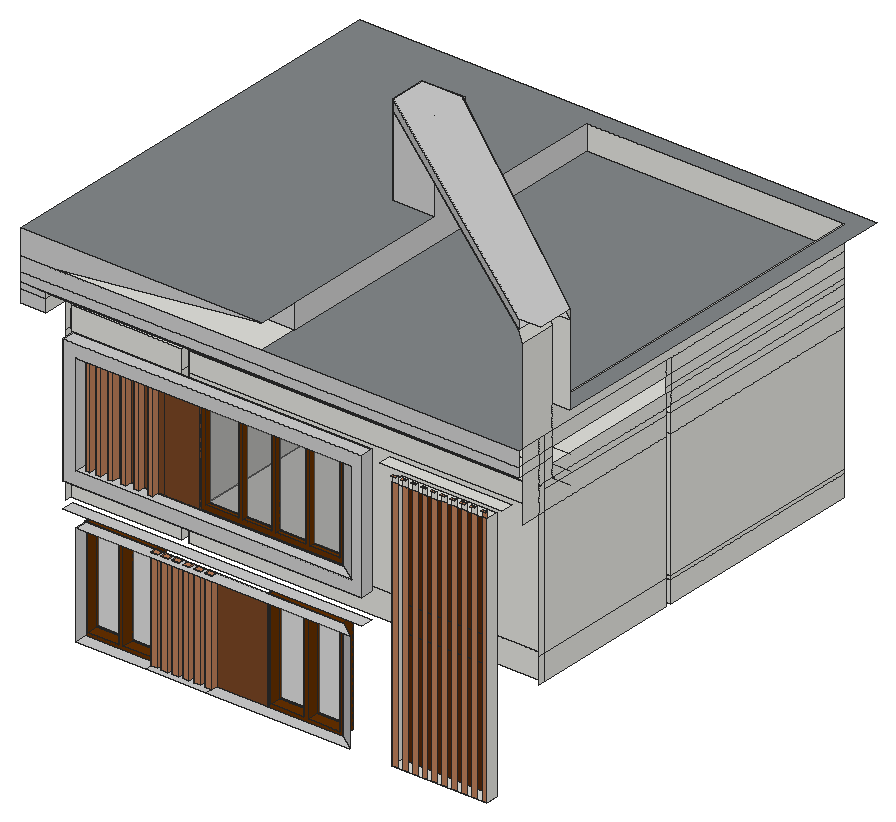
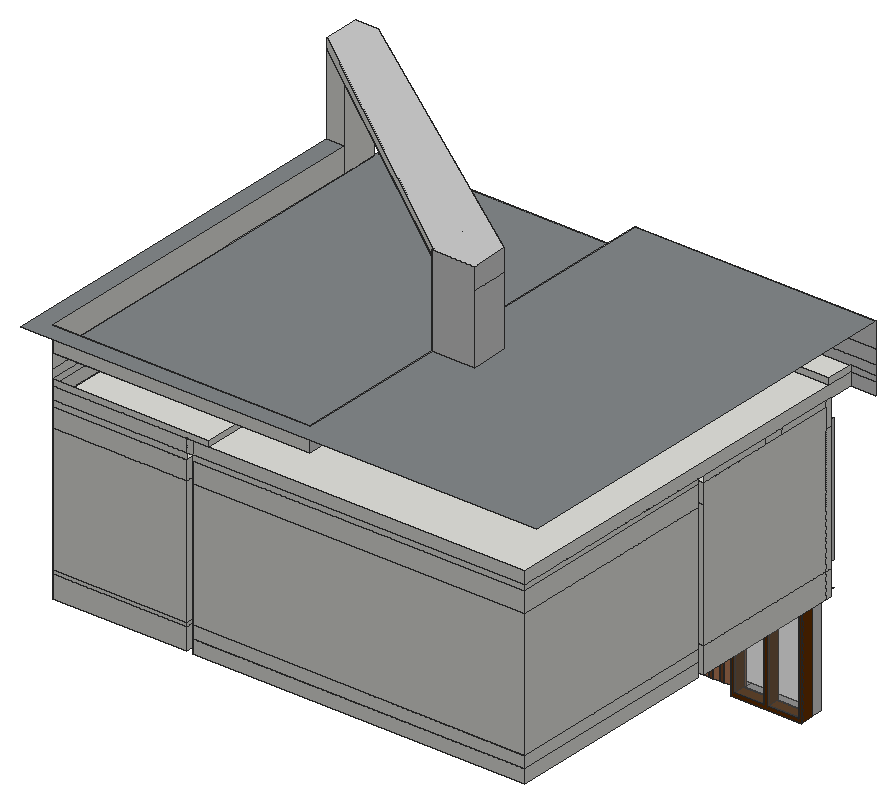
# SketchUp Ruby script. Lengths in inches.
U = 1.inch
M = Sketchup.active_model
def pt(a) = Geom::Point3d.new(a.map { |v| v * U })
def face(e, loops, mat)
  f = e.add_face(loops[0].map { |a| pt(a) })
  loops[1..].each { |l| e.add_face(l.map { |a| pt(a) }).erase! }
  f.material = f.back_material = mat if mat
  f
end
# faces: each face lists its corners as indices into pts; further lists are holes
def faces(e, pts, list, mat = nil) = list.each { |f| face(e, (f[0].is_a?(Array) ? f : [f]).map { |l| l.map { |i| pts[i] } }, mat) }
# xy, xz, yz: faces in a plane at the given z, y or x. An outline is a flat list of corners, or four numbers for a rectangle; further outlines are holes
def ring(l) = l.size == 4 ? [[l[0], l[1]], [l[2], l[1]], [l[2], l[3]], [l[0], l[3]]] : l.each_slice(2).to_a
def flat(e, list, mat, &to3) = list.each { |f| face(e, (f[0].is_a?(Array) ? f : [f]).map { |l| ring(l).map { |u, v| to3.(u, v) } }, mat) }
def xy(e, z, list, mat = nil) = flat(e, list, mat) { |x, y| [x, y, z] }
def xz(e, y, list, mat = nil) = flat(e, list, mat) { |x, z| [x, y, z] }
def yz(e, x, list, mat = nil) = flat(e, list, mat) { |y, z| [x, y, z] }
def lines(e, pts, list) = list.each { |a, b| e.add_line(pt(pts[a]), pt(pts[b])) }
# prism: a flat outline (further loops are holes) pulled along v
def prism(e, loops, v, mat = nil)
  f = face(e, loops, mat); d = Geom::Vector3d.new(v.map { |x| x * U })
  f.pushpull(f.normal.samedirection?(d) ? d.length : -d.length)
end
def box(e, o, s, mat = nil) = prism(e, [[o, [o[0] + s[0], o[1], o[2]], [o[0] + s[0], o[1] + s[1], o[2]], [o[0], o[1] + s[1], o[2]]]], [0, 0, s[2]], mat)
def at(x, y, z, deg = 0) = Geom::Transformation.translation(pt([x, y, z])) * Geom::Transformation.rotation(ORIGIN, Z_AXIS, deg.degrees)
def axes(o, x, y, z) = Geom::Transformation.new([*x, 0, *y, 0, *z, 0, *pt(o).to_a, 1])
def part(name) = M.definitions.add(name)
# library, detail: a bought-in or finely detailed component or shape, given as its bounding box
def library(name, o, s) = part(name).tap { |d| box(d.entities, o, s) }
def detail(e, o, s) = box(e.add_group.entities, o, s)
def put(e, d, t, mat = nil) = e.add_instance(d, t).tap { |i| i.material = mat if mat }
def group(e, t, mat = nil) = e.add_group.tap { |g| g.transformation = t; g.material = mat if mat }.entities
root = M.entities
M.materials.add("[Blacktop Old 01]").color = [132, 136, 139]
M.materials.add("[Brick Antique 01]").color = [88, 41, 11]
M.materials.add("[Carrera Marble]").color = [207, 207, 207]
M.materials.add("[Color A08]").color = [102, 48, 0]
M.materials.add("[Translucent Glass Gray]").color = [128, 128, 128]
M.materials["[Translucent Glass Gray]"].alpha = 0.5
M.materials.add("[Wood Veneer 01]").color = [120, 70, 37]
M.materials.add("[Wood Veneer 02]").color = [190, 128, 91]
c1 = part("Group\#1")
xy(c1.entities,0,[[0,0,125.5,0.3125],[0,0.3125,125.5,4]],"[Color A08]")
xy(c1.entities,4.91,[[4.91,0,60.47,0.3125],[60.47,0,67.75,0.3125],[67.75,0,120.59,0.3125],[4.91,0.3125,60.47,4],[60.47,0.3125,67.75,4],
  [67.75,0.3125,120.59,4]],"[Color A08]")
xy(c1.entities,153.9,[[4.91,0,60.47,0.3125],[67.75,0,120.59,0.3125],[4.91,0.3125,60.47,4],[67.75,0.3125,120.59,4]],"[Color A08]")
xy(c1.entities,158.8125,[[0,0,125.5,0.3125],[0,0.3125,125.5,4]],"[Color A08]")
xz(c1.entities,0,[[[0,0,125.5,158.8125],[4.91,4.91,4.91,153.9,60.47,153.9,60.47,4.91,67.75,4.91,67.75,153.9,120.59,153.9,120.59,4.91]]],"[Color A08]")
xz(c1.entities,0,[[4.91,4.91,60.47,153.9],[67.75,4.91,120.59,153.9]],"[Translucent Glass Gray]")
xz(c1.entities,0.3125,[[[0,0,125.5,158.8125],[4.91,4.91,4.91,153.9,60.47,153.9,60.47,4.91,67.75,4.91,67.75,153.9,120.59,153.9,120.59,4.91]]],"[Color A08]")
xz(c1.entities,4,[[[0,0,125.5,158.8125],[4.91,4.91,4.91,153.9,60.47,153.9,60.47,4.91,67.75,4.91,67.75,153.9,120.59,153.9,120.59,4.91]]],"[Color A08]")
yz(c1.entities,0,[[0,0,0.3125,158.8125],[0.3125,0,4,158.8125]],"[Color A08]")
yz(c1.entities,4.91,[[0,4.91,0.3125,153.9],[0.3125,4.91,4,153.9]],"[Color A08]")
yz(c1.entities,60.47,[[0,4.91,0.3125,153.9],[0.3125,4.91,4,153.9]],"[Color A08]")
yz(c1.entities,67.75,[[0,4.91,0.3125,153.9],[0.3125,4.91,4,153.9]],"[Color A08]")
yz(c1.entities,120.59,[[0,4.91,0.3125,153.9],[0.3125,4.91,4,153.9]],"[Color A08]")
yz(c1.entities,125.5,[[0,0,0.3125,158.8125],[0.3125,0,4,158.8125]],"[Color A08]")
xy(root,441,[[341.75,90.75,431.1875,102.75],[43.25,102.75,108.92,108.75],[215.87,102.75,285.875,108.75]])
xy(root,441,[[43.25,90.75,108.92,102.75],[108.92,90.75,166.36,90.75,166.36,96.875,159.8,96.875,159.8,102.75,155.92,102.75,155.92,96.875,149.36,96.875,149.36,102.75,145.48,102.75,145.48,96.875,138.92,96.875,138.92,102.75,135.23,102.75,135.23,96.875,128.67,96.875,128.67,102.75,125.36,102.75,125.36,96.875,118.8,96.875,118.8,102.75,115.48,102.75,115.48,96.875,108.92,96.875],[166.36,90.75,301.84,90.75,285.875,102.75,166.36,102.75]],"[Carrera Marble]")
xy(root,441,[[108.92,96.875,115.48,102.75],[118.8,96.875,125.36,102.75],[128.67,96.875,135.23,102.75],[138.92,96.875,145.48,102.75],[149.36,96.875,155.92,102.75],
  [159.8,96.875,166.36,102.75]],"[Wood Veneer 02]")
xy(root,537,[[43.25,102.75,108.92,108.75],[215.87,102.75,285.875,108.75]])
xy(root,537,[[43.25,90.75,43.25,102.75,108.92,102.75,108.92,96.875,115.48,96.875,115.48,102.75,118.8,102.75,118.8,96.875,125.36,96.875,125.36,102.75,128.67,102.75,128.67,96.875,135.23,96.875,135.23,102.75,138.92,102.75,138.92,96.875,145.48,96.875,145.48,102.75,149.36,102.75,149.36,96.875,155.92,96.875,155.92,102.75,159.8,102.75,159.8,96.875,166.36,96.875,166.36,102.75,285.875,102.75,301.84,90.75]],"[Carrera Marble]")
xy(root,537,[[108.92,96.875,115.48,102.75],[118.8,96.875,125.36,102.75],[128.67,96.875,135.23,102.75],[138.92,96.875,145.48,102.75],[149.36,96.875,155.92,102.75],
  [159.8,96.875,166.36,102.75]],"[Wood Veneer 02]")
xy(root,549,[[31.25,90.75,312.9375,102.75]],"[Carrera Marble]")
xy(root,561.75,[[24.5,258.8125,337.8125,463]])
xy(root,569.625,[[343.8125,258.8125,470.5,463]])
xy(root,573,[[24.5,108.75,129.23,252.8125],[135.23,108.75,470.5,252.8125],[24.5,258.8125,337.8125,463],[343.8125,258.8125,470.5,463]])
xy(root,573,[[31.25,90.75,312.9375,102.75]],"[Carrera Marble]")
xy(root,585,[[150.42,102.75,285.875,108.75]])
xy(root,585,[[43.25,90.75,304.01,90.75,285.875,102.75,111.29,102.75,111.29,96.0625,106.64,96.0625,106.64,102.75,98.03,102.75,98.03,96.0625,93.38,96.0625,93.38,102.75,85.91,102.75,85.91,96.0625,81.26,96.0625,81.26,102.75,74.22,102.75,74.22,96.0625,69.57,96.0625,69.57,102.75,62.82,102.75,62.82,96.0625,58.17,96.0625,58.17,102.75,52.63,102.75,52.63,96.0625,47.98,96.0625,47.98,102.75,43.25,102.75]],"[Carrera Marble]")
xy(root,585,[[47.98,96.0625,52.63,102.75],[58.17,96.0625,62.82,102.75],[69.57,96.0625,74.22,102.75],[81.26,96.0625,85.91,102.75],[93.38,96.0625,98.03,102.75],
  [106.64,96.0625,111.29,102.75]],"[Wood Veneer 02]")
xy(root,681,[[341.75,90.75,431.1875,102.75]])
xy(root,681,[[43.25,90.75,43.25,102.75,47.98,102.75,47.98,96.0625,52.63,96.0625,52.63,102.75,58.17,102.75,58.17,96.0625,62.82,96.0625,62.82,102.75,69.57,102.75,69.57,96.0625,74.22,96.0625,74.22,102.75,81.26,102.75,81.26,96.0625,85.91,96.0625,85.91,102.75,93.38,102.75,93.38,96.0625,98.03,96.0625,98.03,102.75,106.64,102.75,106.64,96.0625,111.29,96.0625,111.29,102.75,116.8,102.75,116.8,90.75],[116.8,90.75,150.42,102.75],[150.42,90.75,150.42,102.75,285.875,102.75,304.01,90.75],[150.42,102.75,285.875,108.75]],"[Carrera Marble]")
xy(root,681,[[47.98,96.0625,52.63,102.75],[58.17,96.0625,62.82,102.75],[69.57,96.0625,74.22,102.75],[81.26,96.0625,85.91,102.75],[93.38,96.0625,98.03,102.75],
  [106.64,96.0625,111.29,102.75]],"[Wood Veneer 02]")
xy(root,687.5,[[342.74,88.5,347.3,90.75],[351.99,88.5,356.55,90.75],[361.24,88.5,365.8,90.75],[370.49,88.5,375.05,90.75],[379.74,88.5,384.3,90.75],
  [388.99,88.5,393.55,90.75],[398.24,88.5,402.8,90.75],[407.49,88.5,412.05,90.75],[416.93,88.5,421.49,90.75],[427.11,88.5,431.68,90.75]],"[Wood Veneer 02]")
xy(root,693,[[330,90.75,445.6875,102.75]])
xy(root,693,[[31.25,90.75,312.9375,102.75]],"[Carrera Marble]")
xy(root,711,[[24.5,108.75,129.23,252.8125],[343.8125,258.8125,470.5,463]])
xy(root,712,[[24.5,258.8125,337.8125,463]])
xy(root,717,[[24.5,102.75,470.5,463]])
xy(root,729,[[24.5,104.5625,322.875,463]])
xy(root,734.5625,[[24.5,79.3125,470.5,104.5625]])
xy(root,757.1875,[[28.65,79.3125,227.63,118.3125]])
xy(root,757.1875,[[227.63,79.3125,470.5,463]],"[Blacktop Old 01]")
xy(root,780.4375,[[0,79.3125,227.63,79.3125,227.63,283.73,187.76,283.73,187.76,318.86,227.63,318.86,227.63,463,470.5,463,470.5,118.83,487.5,118.83,487.5,480,0,480]],"[Blacktop Old 01]")
xy(root,856.375,[[466.875,83.875,187.76,283.73,227.63,283.73,227.63,316.62,487.5,118.83,466.875,118.83]],"[Carrera Marble]")
xy(root,865.9375,[[466.875,83.875,487.5,83.875,487.5,118.83,227.63,316.62,227.63,318.86,187.76,318.86,187.76,283.73]],"[Carrera Marble]")
xz(root,79.3125,[[0,717,24.5,729],[0,729,24.5,734.5625],[0,734.5625,470.5,743.3125],[0,743.3125,470.5,757.1875],[0,757.1875,28.65,757.1875,227.63,780.4375,0,780.4375]],"[Carrera Marble]")
xz(root,90.75,[[342.74,681,347.3,687.5],[351.99,681,356.55,687.5],[361.24,681,365.8,687.5],[370.49,681,375.05,687.5],[379.74,681,384.3,687.5],
  [388.99,681,393.55,687.5],[398.24,681,402.8,687.5],[407.49,681,412.05,687.5],[416.93,681,421.49,687.5]])
xz(root,90.75,[[[31.25,573,312.9375,693],[43.25,585,304.01,681]]],"[Carrera Marble]")
xz(root,90.75,[[342.74,441,347.3,681],[351.99,441,356.55,681],[361.24,441,365.8,681],[370.49,441,375.05,681],[379.74,441,384.3,681],
  [388.99,441,393.55,681],[398.24,441,402.8,681],[407.49,441,412.05,681],[416.93,441,421.49,681],[427.11,441,431.1875,681],
  [427.11,681,431.1875,687.5]],"[Wood Veneer 02]")
xz(root,96.0625,[[47.98,585,52.63,681],[58.17,585,62.82,681],[69.57,585,74.22,681],[81.26,585,85.91,681],[93.38,585,98.03,681],
  [106.64,585,111.29,681]],"[Wood Veneer 02]")
xz(root,96.875,[[108.92,441,115.48,537],[118.8,441,125.36,537],[128.67,441,135.23,537],[138.92,441,145.48,537],[149.36,441,155.92,537],
  [159.8,441,166.36,537]],"[Wood Veneer 02]")
xz(root,102.75,[[[31.25,573,312.9375,693],[43.25,585,285.875,681]]])
xz(root,102.75,[[341.75,441,431.1875,549],[341.75,549,431.1875,573],[341.75,573,431.1875,681]],"[Brick Antique 01]")
xz(root,102.75,[[115.48,441,118.8,537],[125.36,441,128.67,537],[135.23,441,138.92,537],[145.48,441,149.36,537],[155.92,441,159.8,537],
  [166.36,441,215.87,537],[43.25,585,47.98,681],[52.63,585,58.17,681],[62.82,585,69.57,681],[74.22,585,81.26,681],
  [85.91,585,93.38,681],[98.03,585,106.64,681],[111.29,585,116.8,681],[116.8,585,150.42,681]],"[Wood Veneer 01]")
xz(root,102.75,[[108.92,441,115.48,537],[118.8,441,125.36,537],[128.67,441,135.23,537],[138.92,441,145.48,537],[149.36,441,155.92,537],
  [159.8,441,166.36,537],[47.98,585,52.63,681],[58.17,585,62.82,681],[69.57,585,74.22,681],[81.26,585,85.91,681],
  [93.38,585,98.03,681],[106.64,585,111.29,681]],"[Wood Veneer 02]")
xz(root,104.5625,[[24.5,729,322.875,734.5625]])
xz(root,108.75,[[24.5,549,129.23,573],[135.23,549,470.5,573],[24.5,573,129.23,711],[[135.23,573,470.5,693],[150.42,585,285.875,681]],[135.23,693,470.5,711]])
xz(root,118.3125,[[28.65,757.1875,227.63,757.1875,227.63,780.4375]],"[Carrera Marble]")
xz(root,118.83,[[470.5,780.4375,470.5,845.4375,466.875,856.375,487.5,856.375,487.5,780.4375]])
xz(root,252.8125,[[24.5,549,129.23,573],[135.23,549,470.5,573],[24.5,573,129.23,693],[135.23,573,470.5,693],[24.5,693,129.23,711]])
xz(root,258.8125,[[24.5,549,337.8125,561.75],[343.8125,549,470.5,569.625],[24.5,561.75,252.45,573],[252.45,561.75,260.7,573],[260.7,561.75,337.8125,573],
  [343.8125,569.625,439.36,573],[439.36,569.625,454.49,573],[454.49,569.625,470.5,573],[24.5,573,337.8125,693],[343.8125,573,470.5,693],
  [24.5,693,337.8125,712],[343.8125,693,470.5,711]])
xz(root,283.73,[[187.76,780.4375,227.63,856.375]],"[Carrera Marble]")
xz(root,318.86,[[187.76,780.4375,227.63,865.9375]],"[Carrera Marble]")
xz(root,463,[[24.5,549,337.8125,561.75],[343.8125,549,470.5,569.625],[24.5,561.75,337.8125,573],[343.8125,569.625,470.5,573],[24.5,573,337.8125,693],
  [343.8125,573,470.5,693],[24.5,693,337.8125,712],[343.8125,693,470.5,711],[343.8125,711,470.5,717],[24.5,712,337.8125,717],
  [24.5,717,337.8125,729],[337.8125,717,343.8125,729],[343.8125,717,470.5,729],[322.875,729,470.5,734.5625],[227.63,757.1875,470.5,780.4375]])
yz(root,24.5,[[102.75,549,108.75,573],[108.75,549,252.8125,573],[258.8125,549,463,561.75],[258.8125,561.75,463,573],[102.75,573,108.75,693],
  [108.75,573,252.8125,711],[258.8125,573,463,693],[102.75,693,108.75,717],[258.8125,693,463,712],[108.75,711,160.04,717],
  [160.04,711,180.78,717],[180.78,711,252.8125,717],[258.8125,712,463,717],[79.3125,717,463,729],[79.3125,729,104.5625,734.5625]])
yz(root,31.25,[[90.75,573,102.75,693]],"[Carrera Marble]")
yz(root,43.25,[[90.75,441,102.75,537],[102.75,441,108.75,537],[90.75,585,102.75,681]],"[Carrera Marble]")
yz(root,47.98,[[96.0625,585,102.75,681]],"[Wood Veneer 02]")
yz(root,52.63,[[96.0625,585,102.75,681]],"[Wood Veneer 02]")
yz(root,58.17,[[96.0625,585,102.75,681]],"[Wood Veneer 02]")
yz(root,62.82,[[96.0625,585,102.75,681]],"[Wood Veneer 02]")
yz(root,69.57,[[96.0625,585,102.75,681]],"[Wood Veneer 02]")
yz(root,74.22,[[96.0625,585,102.75,681]],"[Wood Veneer 02]")
yz(root,81.26,[[96.0625,585,102.75,681]],"[Wood Veneer 02]")
yz(root,85.91,[[96.0625,585,102.75,681]],"[Wood Veneer 02]")
yz(root,93.38,[[96.0625,585,102.75,681]],"[Wood Veneer 02]")
yz(root,98.03,[[96.0625,585,102.75,681]],"[Wood Veneer 02]")
yz(root,106.64,[[96.0625,585,102.75,681]],"[Wood Veneer 02]")
yz(root,108.92,[[102.75,441,108.75,537]],"[Wood Veneer 01]")
yz(root,108.92,[[96.875,441,102.75,537]],"[Wood Veneer 02]")
yz(root,111.29,[[96.0625,585,102.75,681]],"[Wood Veneer 02]")
yz(root,115.48,[[96.875,441,102.75,537]],"[Wood Veneer 02]")
yz(root,118.8,[[96.875,441,102.75,537]],"[Wood Veneer 02]")
yz(root,125.36,[[96.875,441,102.75,537]],"[Wood Veneer 02]")
yz(root,128.67,[[96.875,441,102.75,537]],"[Wood Veneer 02]")
yz(root,129.23,[[108.75,549,252.8125,573],[108.75,573,252.8125,693],[108.75,693,252.8125,711]])
yz(root,135.23,[[108.75,549,252.8125,573],[108.75,573,252.8125,693],[108.75,693,252.8125,711]])
yz(root,135.23,[[96.875,441,102.75,537]],"[Wood Veneer 02]")
yz(root,138.92,[[96.875,441,102.75,537]],"[Wood Veneer 02]")
yz(root,145.48,[[96.875,441,102.75,537]],"[Wood Veneer 02]")
yz(root,149.36,[[96.875,441,102.75,537]],"[Wood Veneer 02]")
yz(root,150.42,[[102.75,585,108.75,681]],"[Wood Veneer 01]")
yz(root,155.92,[[96.875,441,102.75,537]],"[Wood Veneer 02]")
yz(root,159.8,[[96.875,441,102.75,537]],"[Wood Veneer 02]")
yz(root,166.36,[[96.875,441,102.75,537]],"[Wood Veneer 02]")
yz(root,187.76,[[283.73,780.4375,318.86,845.4375],[283.73,845.4375,318.86,865.9375]],"[Carrera Marble]")
yz(root,215.87,[[102.75,441,108.75,537]],"[Wood Veneer 01]")
yz(root,227.63,[[118.3125,757.1875,463,757.1875,463,780.4375,318.86,780.4375,318.86,865.9375,316.62,865.9375,316.62,856.375,283.73,856.375,283.73,780.4375,118.3125,780.4375]],"[Carrera Marble]")
yz(root,285.875,[[102.75,441,108.75,537],[102.75,585,108.75,681]],"[Carrera Marble]")
yz(root,312.9375,[[90.75,573,102.75,693]],"[Carrera Marble]")
yz(root,322.875,[[104.5625,729,463,734.5625]])
yz(root,337.8125,[[258.8125,549,463,561.75],[258.8125,561.75,463,573],[258.8125,573,463,693],[258.8125,693,463,712]])
yz(root,341.75,[[90.75,441,102.75,681]])
yz(root,343.8125,[[258.8125,549,463,569.625],[258.8125,569.625,463,573],[258.8125,573,463,693],[258.8125,693,463,711]])
yz(root,431.1875,[[90.75,441,102.75,681]])
yz(root,470.5,[[102.75,549,108.75,573],[108.75,549,252.8125,573],[258.8125,549,463,569.625],[258.8125,569.625,463,573],[102.75,573,108.75,693],
  [108.75,573,252.8125,693],[258.8125,573,463,693],[83.875,693,102.75,734.5625],[102.75,693,108.75,717],[108.75,693,252.8125,711],
  [258.8125,693,463,711],[108.75,711,252.8125,717],[258.8125,711,463,717],[102.75,717,108.75,734.5625],[108.75,717,118.83,734.5625],
  [118.83,717,252.8125,729],[252.8125,717,258.8125,729],[258.8125,717,463,729],[252.8125,729,258.8125,734.5625],[258.8125,729,463,734.5625],
  [83.875,734.5625,102.75,743.3125],[102.75,734.5625,108.75,743.3125],[108.75,734.5625,118.83,743.3125],[252.8125,734.5625,258.8125,743.3125],[258.8125,734.5625,463,743.3125],
  [83.875,743.3125,102.75,757.1875],[102.75,743.3125,108.75,757.1875],[108.75,743.3125,118.83,757.1875],[118.83,743.3125,252.8125,757.1875],[252.8125,743.3125,258.8125,757.1875],
  [258.8125,743.3125,463,757.1875],[83.875,757.1875,118.83,845.4375],[118.83,757.1875,463,780.4375]])
p = [[301.84,90.75,441],[301.84,90.75,537],[285.875,102.75,537],[285.875,102.75,441],[304.01,90.75,681],[285.875,102.75,681],
  [285.875,102.75,585],[304.01,90.75,585],[227.63,79.3125,780.4375],[28.65,79.3125,757.1875],[28.65,118.3125,757.1875],[227.63,118.3125,780.4375],
  [470.5,83.875,845.4375],[466.875,83.875,856.375],[466.875,118.83,856.375],[470.5,118.83,845.4375],[187.76,283.73,856.375],[466.875,83.875,865.9375],
  [187.76,283.73,865.9375],[487.5,118.83,856.375],[227.63,316.62,856.375],[227.63,316.62,865.9375],[487.5,118.83,865.9375],[129.23,252.8125,711],
  [129.23,252.8125,717],[149.36,252.8125,717],[149.36,252.8125,711],[135.23,252.8125,711],[135.23,252.8125,717],[135.23,108.75,711],
  [135.23,108.75,717],[56.125,258.8125,717],[56.125,258.8125,712],[337.8125,258.8125,712],[337.8125,258.8125,717],[358.375,258.8125,717],
  [358.375,258.8125,711],[343.8125,258.8125,711],[343.8125,258.8125,717],[470.5,252.8125,711],[431.48,100.49,441],[431.48,93.99,441],
  [470.5,118.83,717],[487.5,118.83,717],[470.5,118.83,729],[487.5,118.83,729],[470.5,118.83,743.3125],[487.5,118.83,743.3125],
  [470.5,79.3125,743.3125],[470.5,83.875,743.3125],[227.49,283.73,845.4375],[227.63,283.73,845.4375],[227.49,283.73,856.375],[227.49,283.73,865.9375]]
faces(root,p,[[0,1,2,3],[4,5,6,7],[8,9,10,11],[16,13,17,18]],"[Carrera Marble]")
faces(root,p,[[12,13,14,15],[19,20,21,22]])
lines(root,p,[[23,24],[25,26],[27,28],[29,30],[31,32],[33,34],[35,36],[37,38],[26,39],[40,41],[42,43],[44,45],
  [46,47],[48,49],[50,51],[52,53]])
put(root,c1,axes([42.11,114.75,441],[0.53236,0,0],[0,-3,0],[0,0,0.60449]))
put(root,c1,axes([215.06,114.75,441],[0.5643,0,0],[0,-3,0],[0,0,0.60449]))
g1 = group(root,at(150.42,109.2,585))
xy(g1,0,[[0,-4.7,135.46,-0.28],[0,-0.28,135.46,0]],"[Color A08]")
xy(g1,4.65,[[5.01,-4.7,35.46,-0.28],[35.46,-4.7,39.58,-0.28],[39.58,-4.7,66.59,-0.28],[66.59,-4.7,70.72,-0.28],[70.72,-4.7,98.8125,-0.28],
  [98.8125,-4.7,102.94,-0.28],[102.94,-4.7,131.33,-0.28],[5.01,-0.28,35.46,0],[35.46,-0.28,39.58,0],[39.58,-0.28,66.59,0],
  [66.59,-0.28,70.72,0],[70.72,-0.28,98.8125,0],[98.8125,-0.28,102.94,0],[102.94,-0.28,131.33,0]],"[Color A08]")
xy(g1,91.35,[[5.01,-4.7,35.46,-0.28],[39.58,-4.7,66.59,-0.28],[70.72,-4.7,98.8125,-0.28],[102.94,-4.7,131.33,-0.28],[5.01,-0.28,35.46,0],
  [39.58,-0.28,66.59,0],[70.72,-0.28,98.8125,0],[102.94,-0.28,131.33,0]],"[Color A08]")
xy(g1,96,[[0,-4.7,135.46,-0.28],[0,-0.28,135.46,0]],"[Color A08]")
xz(g1,-4.7,[[[0,0,135.46,96],[5.01,4.65,5.01,91.35,35.46,91.35,35.46,4.65,39.58,4.65,39.58,91.35,66.59,91.35,66.59,4.65,70.72,4.65,70.72,91.35,98.8125,91.35,98.8125,4.65,102.94,4.65,102.94,91.35,131.33,91.35,131.33,4.65]]],"[Color A08]")
xz(g1,-0.28,[[[0,0,135.46,96],[5.01,4.65,5.01,91.35,35.46,91.35,35.46,4.65,39.58,4.65,39.58,91.35,66.59,91.35,66.59,4.65,70.72,4.65,70.72,91.35,98.8125,91.35,98.8125,4.65,102.94,4.65,102.94,91.35,131.33,91.35,131.33,4.65]]],"[Color A08]")
xz(g1,0,[[[0,0,135.46,96],[5.01,4.65,5.01,91.35,35.46,91.35,35.46,4.65,39.58,4.65,39.58,91.35,66.59,91.35,66.59,4.65,70.72,4.65,70.72,91.35,98.8125,91.35,98.8125,4.65,102.94,4.65,102.94,91.35,131.33,91.35,131.33,4.65]]],"[Color A08]")
xz(g1,0,[[5.01,4.65,35.46,91.35],[39.58,4.65,66.59,91.35],[70.72,4.65,98.8125,91.35],[102.94,4.65,131.33,91.35]],"[Translucent Glass Gray]")
yz(g1,0,[[-4.7,0,-0.28,96],[-0.28,0,0,96]],"[Color A08]")
yz(g1,5.01,[[-4.7,4.65,-0.28,91.35],[-0.28,4.65,0,91.35]],"[Color A08]")
yz(g1,35.46,[[-4.7,4.65,-0.28,91.35],[-0.28,4.65,0,91.35]],"[Color A08]")
yz(g1,39.58,[[-4.7,4.65,-0.28,91.35],[-0.28,4.65,0,91.35]],"[Color A08]")
yz(g1,66.59,[[-4.7,4.65,-0.28,91.35],[-0.28,4.65,0,91.35]],"[Color A08]")
yz(g1,70.72,[[-4.7,4.65,-0.28,91.35],[-0.28,4.65,0,91.35]],"[Color A08]")
yz(g1,98.8125,[[-4.7,4.65,-0.28,91.35],[-0.28,4.65,0,91.35]],"[Color A08]")
yz(g1,102.94,[[-4.7,4.65,-0.28,91.35],[-0.28,4.65,0,91.35]],"[Color A08]")
yz(g1,131.33,[[-4.7,4.65,-0.28,91.35],[-0.28,4.65,0,91.35]],"[Color A08]")
yz(g1,135.46,[[-4.7,0,-0.28,96],[-0.28,0,0,96]],"[Color A08]")
